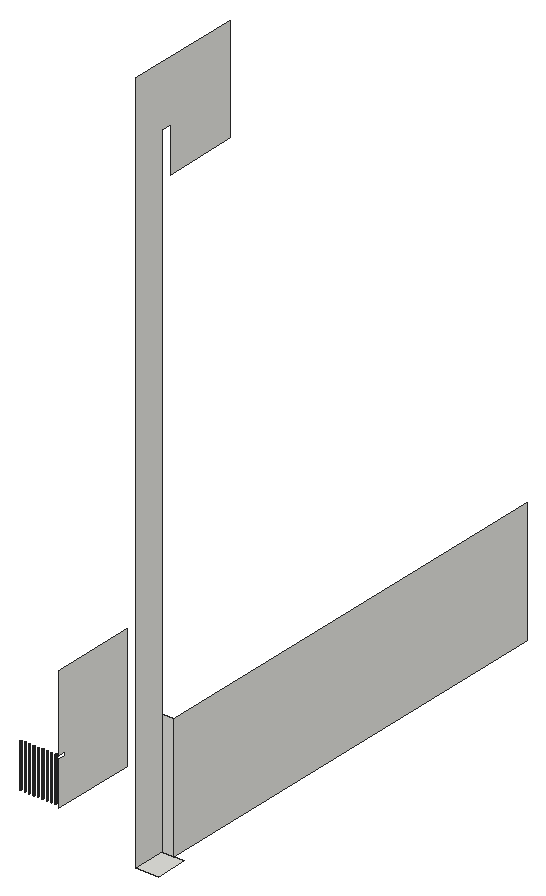
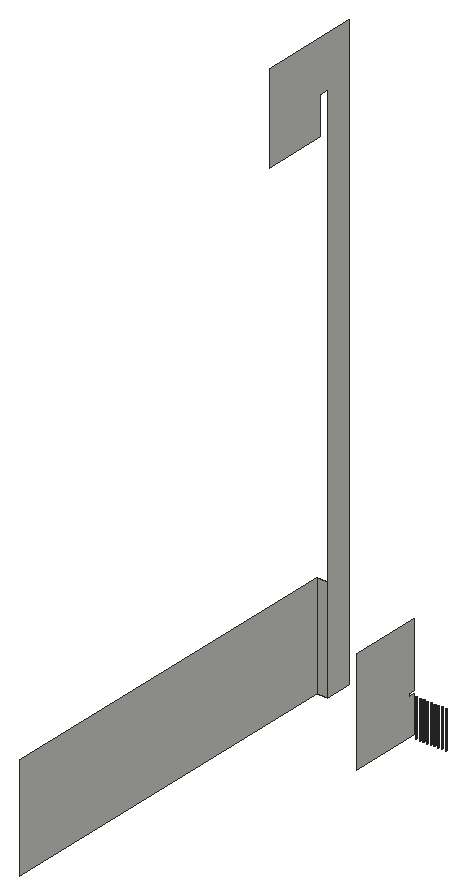
# SketchUp Ruby script. Lengths in inches.
U = 1.inch
M = Sketchup.active_model
def pt(a) = Geom::Point3d.new(a.map { |v| v * U })
def face(e, loops, mat)
  f = e.add_face(loops[0].map { |a| pt(a) })
  loops[1..].each { |l| e.add_face(l.map { |a| pt(a) }).erase! }
  f.material = f.back_material = mat if mat
  f
end
# faces: each face lists its corners as indices into pts; further lists are holes
def faces(e, pts, list, mat = nil) = list.each { |f| face(e, (f[0].is_a?(Array) ? f : [f]).map { |l| l.map { |i| pts[i] } }, mat) }
# xy, xz, yz: faces in a plane at the given z, y or x. An outline is a flat list of corners, or four numbers for a rectangle; further outlines are holes
def ring(l) = l.size == 4 ? [[l[0], l[1]], [l[2], l[1]], [l[2], l[3]], [l[0], l[3]]] : l.each_slice(2).to_a
def flat(e, list, mat, &to3) = list.each { |f| face(e, (f[0].is_a?(Array) ? f : [f]).map { |l| ring(l).map { |u, v| to3.(u, v) } }, mat) }
def xy(e, z, list, mat = nil) = flat(e, list, mat) { |x, y| [x, y, z] }
def xz(e, y, list, mat = nil) = flat(e, list, mat) { |x, z| [x, y, z] }
def yz(e, x, list, mat = nil) = flat(e, list, mat) { |y, z| [x, y, z] }
def lines(e, pts, list) = list.each { |a, b| e.add_line(pt(pts[a]), pt(pts[b])) }
# prism: a flat outline (further loops are holes) pulled along v
def prism(e, loops, v, mat = nil)
  f = face(e, loops, mat); d = Geom::Vector3d.new(v.map { |x| x * U })
  f.pushpull(f.normal.samedirection?(d) ? d.length : -d.length)
end
def box(e, o, s, mat = nil) = prism(e, [[o, [o[0] + s[0], o[1], o[2]], [o[0] + s[0], o[1] + s[1], o[2]], [o[0], o[1] + s[1], o[2]]]], [0, 0, s[2]], mat)
def at(x, y, z, deg = 0) = Geom::Transformation.translation(pt([x, y, z])) * Geom::Transformation.rotation(ORIGIN, Z_AXIS, deg.degrees)
def axes(o, x, y, z) = Geom::Transformation.new([*x, 0, *y, 0, *z, 0, *pt(o).to_a, 1])
def part(name) = M.definitions.add(name)
# library, detail: a bought-in or finely detailed component or shape, given as its bounding box
def library(name, o, s) = part(name).tap { |d| box(d.entities, o, s) }
def detail(e, o, s) = box(e.add_group.entities, o, s)
def put(e, d, t, mat = nil) = e.add_instance(d, t).tap { |i| i.material = mat if mat }
def group(e, t, mat = nil) = e.add_group.tap { |g| g.transformation = t; g.material = mat if mat }.entities
root = M.entities
xy(root,204.9375,[[673.48,81.125,703.6875,124.5],[472.27,135.31,472.06,135.34,471.86,135.42,471.69,135.55,471.5625,135.72,471.48,135.91,471.45,136.12,471.48,136.33,471.5625,136.53,471.69,136.7,471.86,136.83,472.06,136.91,472.27,136.93,472.48,136.91,472.67,136.83,472.84,136.7,472.97,136.53,473.05,136.33,473.08,136.12,473.05,135.91,472.97,135.72,472.84,135.55,472.67,135.42,472.48,135.34],[478.27,135.31,478.06,135.34,477.86,135.42,477.69,135.55,477.5625,135.72,477.48,135.91,477.45,136.12,477.48,136.33,477.5625,136.53,477.69,136.7,477.86,136.83,478.06,136.91,478.27,136.93,478.48,136.91,478.67,136.83,478.84,136.7,478.97,136.53,479.05,136.33,479.08,136.12,479.05,135.91,478.97,135.72,478.84,135.55,478.67,135.42,478.48,135.34],[484.2,135.31,483.99,135.34,483.8,135.42,483.63,135.55,483.5,135.72,483.42,135.91,483.39,136.12,483.42,136.33,483.5,136.53,483.63,136.7,483.8,136.83,483.99,136.91,484.2,136.93,484.41,136.91,484.61,136.83,484.78,136.7,484.91,136.53,484.99,136.33,485.02,136.12,484.99,135.91,484.91,135.72,484.78,135.55,484.61,135.42,484.41,135.34],[490.27,135.31,490.06,135.34,489.86,135.42,489.69,135.55,489.5625,135.72,489.48,135.91,489.45,136.12,489.48,136.33,489.5625,136.53,489.69,136.7,489.86,136.83,490.06,136.91,490.27,136.93,490.48,136.91,490.67,136.83,490.84,136.7,490.97,136.53,491.05,136.33,491.08,136.12,491.05,135.91,490.97,135.72,490.84,135.55,490.67,135.42,490.48,135.34],
  [496.27,135.31,496.06,135.34,495.86,135.42,495.69,135.55,495.5625,135.72,495.48,135.91,495.45,136.12,495.48,136.33,495.5625,136.53,495.69,136.7,495.86,136.83,496.06,136.91,496.27,136.93,496.48,136.91,496.67,136.83,496.84,136.7,496.97,136.53,497.05,136.33,497.08,136.12,497.05,135.91,496.97,135.72,496.84,135.55,496.67,135.42,496.48,135.34],[502.27,135.31,502.06,135.34,501.86,135.42,501.69,135.55,501.5625,135.72,501.48,135.91,501.45,136.12,501.48,136.33,501.5625,136.53,501.69,136.7,501.86,136.83,502.06,136.91,502.27,136.93,502.48,136.91,502.67,136.83,502.84,136.7,502.97,136.53,503.05,136.33,503.08,136.12,503.05,135.91,502.97,135.72,502.84,135.55,502.67,135.42,502.48,135.34],[508.14,135.31,507.93,135.34,507.74,135.42,507.57,135.55,507.4375,135.72,507.36,135.91,507.33,136.12,507.36,136.33,507.4375,136.53,507.57,136.7,507.74,136.83,507.93,136.91,508.14,136.93,508.35,136.91,508.55,136.83,508.72,136.7,508.85,136.53,508.93,136.33,508.95,136.12,508.93,135.91,508.85,135.72,508.72,135.55,508.55,135.42,508.35,135.34],[514.2,135.31,513.99,135.34,513.8,135.42,513.63,135.55,513.5,135.72,513.42,135.91,513.39,136.12,513.42,136.33,513.5,136.53,513.63,136.7,513.8,136.83,513.99,136.91,514.2,136.93,514.41,136.91,514.61,136.83,514.78,136.7,514.91,136.53,514.99,136.33,515.02,136.12,514.99,135.91,514.91,135.72,514.78,135.55,514.61,135.42,514.41,135.34],[520.27,135.31,520.06,135.34,519.86,135.42,519.69,135.55,519.5625,135.72,519.48,135.91,519.45,136.12,519.48,136.33,519.5625,136.53,519.69,136.7,519.86,136.83,520.06,136.91,520.27,136.93,520.48,136.91,520.67,136.83,520.84,136.7,520.97,136.53,521.05,136.33,521.08,136.12,521.05,135.91,520.97,135.72,520.84,135.55,520.67,135.42,520.48,135.34]])
xz(root,124.5,[[673.48,204.9375,690.4375,372.9375]])
yz(root,528.75,[[130.75,204.9375,130.75,264.83,140.05,264.83,140.05,269.02,130.75,269.02,130.75,372.9375,246,372.9375,246,204.9375]])
yz(root,673.48,[[81.125,204.9375,81.125,1168.125,241.25,1168.125,241.25,1024.6875,139.4375,1024.6875,139.4375,1085.75,124.5,1085.75,124.5,204.9375]])
yz(root,690.4375,[[124.5,204.9375,724.5,372.9375]])
p = [[471.86,135.42,204.9375],[472.06,135.34,204.9375],[472.06,135.34,264.83],[471.86,135.42,264.83],[472.27,135.31,204.9375],[472.27,135.31,264.83],
  [472.48,135.34,204.9375],[472.48,135.34,264.83],[472.67,135.42,204.9375],[472.67,135.42,264.83],[477.86,135.42,204.9375],[478.06,135.34,204.9375],
  [478.06,135.34,264.83],[477.86,135.42,264.83],[478.27,135.31,204.9375],[478.27,135.31,264.83],[478.48,135.34,204.9375],[478.48,135.34,264.83],
  [478.67,135.42,204.9375],[478.67,135.42,264.83],[483.8,135.42,204.9375],[483.99,135.34,204.9375],[483.99,135.34,264.83],[483.8,135.42,264.83],
  [484.2,135.31,204.9375],[484.2,135.31,264.83],[484.41,135.34,204.9375],[484.41,135.34,264.83],[484.61,135.42,204.9375],[484.61,135.42,264.83],
  [489.86,135.42,204.9375],[490.06,135.34,204.9375],[490.06,135.34,264.83],[489.86,135.42,264.83],[490.27,135.31,204.9375],[490.27,135.31,264.83],
  [490.48,135.34,204.9375],[490.48,135.34,264.83],[490.67,135.42,204.9375],[490.67,135.42,264.83],[495.86,135.42,204.9375],[496.06,135.34,204.9375],
  [496.06,135.34,264.83],[495.86,135.42,264.83],[496.27,135.31,204.9375],[496.27,135.31,264.83],[496.48,135.34,204.9375],[496.48,135.34,264.83],
  [496.67,135.42,204.9375],[496.67,135.42,264.83],[501.86,135.42,204.9375],[502.06,135.34,204.9375],[502.06,135.34,264.83],[501.86,135.42,264.83],
  [502.27,135.31,204.9375],[502.27,135.31,264.83],[502.48,135.34,204.9375],[502.48,135.34,264.83],[502.67,135.42,204.9375],[502.67,135.42,264.83],
  [507.74,135.42,204.9375],[507.93,135.34,204.9375],[507.93,135.34,264.83],[507.74,135.42,264.83],[508.14,135.31,204.9375],[508.14,135.31,264.83],
  [508.35,135.34,204.9375],[508.35,135.34,264.83],[508.55,135.42,204.9375],[508.55,135.42,264.83],[513.8,135.42,204.9375],[513.99,135.34,204.9375],
  [513.99,135.34,264.83],[513.8,135.42,264.83],[514.2,135.31,204.9375],[514.2,135.31,264.83],[514.41,135.34,204.9375],[514.41,135.34,264.83],
  [514.61,135.42,204.9375],[514.61,135.42,264.83],[519.86,135.42,204.9375],[520.06,135.34,204.9375],[520.06,135.34,264.83],[519.86,135.42,264.83],
  [520.27,135.31,204.9375],[520.27,135.31,264.83],[520.48,135.34,204.9375],[520.48,135.34,264.83],[520.67,135.42,204.9375],[520.67,135.42,264.83],
  [472.84,135.55,204.9375],[472.84,135.55,264.83],[477.69,135.55,204.9375],[477.69,135.55,264.83],[478.84,135.55,204.9375],[478.84,135.55,264.83],
  [483.63,135.55,204.9375],[483.63,135.55,264.83],[484.78,135.55,204.9375],[484.78,135.55,264.83],[489.69,135.55,204.9375],[489.69,135.55,264.83],
  [490.84,135.55,204.9375],[490.84,135.55,264.83],[495.69,135.55,204.9375],[495.69,135.55,264.83],[496.84,135.55,204.9375],[496.84,135.55,264.83],
  [501.69,135.55,204.9375],[501.69,135.55,264.83],[502.84,135.55,204.9375],[502.84,135.55,264.83],[507.57,135.55,204.9375],[507.57,135.55,264.83],
  [508.72,135.55,204.9375],[508.72,135.55,264.83],[513.63,135.55,204.9375],[513.63,135.55,264.83],[514.78,135.55,204.9375],[514.78,135.55,264.83],
  [519.69,135.55,204.9375],[519.69,135.55,264.83],[520.84,135.55,204.9375],[520.84,135.55,264.83],[472.97,135.72,204.9375],[472.97,135.72,264.83],
  [477.5625,135.72,204.9375],[477.5625,135.72,264.83],[478.97,135.72,204.9375],[478.97,135.72,264.83],[483.5,135.72,204.9375],[483.5,135.72,264.83],
  [484.91,135.72,204.9375],[484.91,135.72,264.83],[489.5625,135.72,204.9375],[489.5625,135.72,264.83],[490.97,135.72,204.9375],[490.97,135.72,264.83],
  [495.5625,135.72,204.9375],[495.5625,135.72,264.83],[496.97,135.72,204.9375],[496.97,135.72,264.83],[501.5625,135.72,204.9375],[501.5625,135.72,264.83],
  [502.97,135.72,204.9375],[502.97,135.72,264.83],[507.4375,135.72,204.9375],[507.4375,135.72,264.83],[508.85,135.72,204.9375],[508.85,135.72,264.83],
  [513.5,135.72,204.9375],[513.5,135.72,264.83],[514.91,135.72,204.9375],[514.91,135.72,264.83],[519.5625,135.72,204.9375],[519.5625,135.72,264.83],
  [520.97,135.72,204.9375],[520.97,135.72,264.83],[473.05,135.91,204.9375],[473.05,135.91,264.83],[477.48,135.91,204.9375],[477.48,135.91,264.83],
  [479.05,135.91,204.9375],[479.05,135.91,264.83],[483.42,135.91,204.9375],[483.42,135.91,264.83],[484.99,135.91,204.9375],[484.99,135.91,264.83],
  [489.48,135.91,204.9375],[489.48,135.91,264.83],[491.05,135.91,204.9375],[491.05,135.91,264.83],[495.48,135.91,204.9375],[495.48,135.91,264.83],
  [497.05,135.91,204.9375],[497.05,135.91,264.83],[501.48,135.91,204.9375],[501.48,135.91,264.83],[503.05,135.91,204.9375],[503.05,135.91,264.83],
  [507.36,135.91,204.9375],[507.36,135.91,264.83],[508.93,135.91,204.9375],[508.93,135.91,264.83],[513.42,135.91,204.9375],[513.42,135.91,264.83],
  [514.99,135.91,204.9375],[514.99,135.91,264.83],[519.48,135.91,204.9375],[519.48,135.91,264.83],[521.05,135.91,204.9375],[521.05,135.91,264.83],
  [473.08,136.12,204.9375],[473.08,136.12,264.83],[477.45,136.12,204.9375],[477.45,136.12,264.83],[479.08,136.12,204.9375],[479.08,136.12,264.83],
  [483.39,136.12,204.9375],[483.39,136.12,264.83],[485.02,136.12,204.9375],[485.02,136.12,264.83],[489.45,136.12,204.9375],[489.45,136.12,264.83],
  [491.08,136.12,204.9375],[491.08,136.12,264.83],[495.45,136.12,204.9375],[495.45,136.12,264.83],[497.08,136.12,204.9375],[497.08,136.12,264.83],
  [501.45,136.12,204.9375],[501.45,136.12,264.83],[503.08,136.12,204.9375],[503.08,136.12,264.83],[507.33,136.12,204.9375],[507.33,136.12,264.83],
  [508.95,136.12,204.9375],[508.95,136.12,264.83],[513.39,136.12,204.9375],[513.39,136.12,264.83],[515.02,136.12,204.9375],[515.02,136.12,264.83],
  [519.45,136.12,204.9375],[519.45,136.12,264.83],[521.08,136.12,204.9375],[521.08,136.12,264.83],[473.05,136.33,204.9375],[473.05,136.33,264.83],
  [477.48,136.33,204.9375],[477.48,136.33,264.83],[479.05,136.33,204.9375],[479.05,136.33,264.83],[483.42,136.33,204.9375],[483.42,136.33,264.83],
  [484.99,136.33,204.9375],[484.99,136.33,264.83],[489.48,136.33,204.9375],[489.48,136.33,264.83],[491.05,136.33,204.9375],[491.05,136.33,264.83],
  [495.48,136.33,204.9375],[495.48,136.33,264.83],[497.05,136.33,204.9375],[497.05,136.33,264.83],[501.48,136.33,204.9375],[501.48,136.33,264.83],
  [503.05,136.33,204.9375],[503.05,136.33,264.83],[507.36,136.33,204.9375],[507.36,136.33,264.83],[508.93,136.33,204.9375],[508.93,136.33,264.83],
  [513.42,136.33,204.9375],[513.42,136.33,264.83],[514.99,136.33,204.9375],[514.99,136.33,264.83],[519.48,136.33,204.9375],[519.48,136.33,264.83],
  [521.05,136.33,204.9375],[521.05,136.33,264.83],[472.97,136.53,204.9375],[472.97,136.53,264.83],[477.5625,136.53,204.9375],[477.5625,136.53,264.83],
  [478.97,136.53,204.9375],[478.97,136.53,264.83],[483.5,136.53,204.9375],[483.5,136.53,264.83],[484.91,136.53,204.9375],[484.91,136.53,264.83],
  [489.5625,136.53,204.9375],[489.5625,136.53,264.83],[490.97,136.53,204.9375],[490.97,136.53,264.83],[495.5625,136.53,204.9375],[495.5625,136.53,264.83],
  [496.97,136.53,204.9375],[496.97,136.53,264.83],[501.5625,136.53,204.9375],[501.5625,136.53,264.83],[502.97,136.53,204.9375],[502.97,136.53,264.83],
  [507.4375,136.53,204.9375],[507.4375,136.53,264.83],[508.85,136.53,204.9375],[508.85,136.53,264.83],[513.5,136.53,204.9375],[513.5,136.53,264.83],
  [514.91,136.53,204.9375],[514.91,136.53,264.83],[519.5625,136.53,204.9375],[519.5625,136.53,264.83],[520.97,136.53,204.9375],[520.97,136.53,264.83],
  [472.84,136.7,204.9375],[472.84,136.7,264.83],[477.69,136.7,204.9375],[477.69,136.7,264.83],[478.84,136.7,204.9375],[478.84,136.7,264.83],
  [483.63,136.7,204.9375],[483.63,136.7,264.83],[484.78,136.7,204.9375],[484.78,136.7,264.83],[489.69,136.7,204.9375],[489.69,136.7,264.83],
  [490.84,136.7,204.9375],[490.84,136.7,264.83],[495.69,136.7,204.9375],[495.69,136.7,264.83],[496.84,136.7,204.9375],[496.84,136.7,264.83],
  [501.69,136.7,204.9375],[501.69,136.7,264.83],[502.84,136.7,204.9375],[502.84,136.7,264.83],[507.57,136.7,204.9375],[507.57,136.7,264.83],
  [508.72,136.7,204.9375],[508.72,136.7,264.83],[513.63,136.7,204.9375],[513.63,136.7,264.83],[514.78,136.7,204.9375],[514.78,136.7,264.83],
  [519.69,136.7,204.9375],[519.69,136.7,264.83],[520.84,136.7,204.9375],[520.84,136.7,264.83],[472.67,136.83,204.9375],[472.67,136.83,264.83],
  [477.86,136.83,204.9375],[477.86,136.83,264.83],[478.67,136.83,204.9375],[478.67,136.83,264.83],[483.8,136.83,204.9375],[483.8,136.83,264.83],
  [484.61,136.83,204.9375],[484.61,136.83,264.83],[489.86,136.83,204.9375],[489.86,136.83,264.83],[490.67,136.83,204.9375],[490.67,136.83,264.83],
  [495.86,136.83,204.9375],[495.86,136.83,264.83],[496.67,136.83,204.9375],[496.67,136.83,264.83],[501.86,136.83,204.9375],[501.86,136.83,264.83],
  [502.67,136.83,204.9375],[502.67,136.83,264.83],[507.74,136.83,204.9375],[507.74,136.83,264.83],[508.55,136.83,204.9375],[508.55,136.83,264.83],
  [513.8,136.83,204.9375],[513.8,136.83,264.83],[514.61,136.83,204.9375],[514.61,136.83,264.83],[519.86,136.83,204.9375],[519.86,136.83,264.83],
  [520.67,136.83,204.9375],[520.67,136.83,264.83],[472.06,136.91,204.9375],[471.86,136.83,204.9375],[471.86,136.83,264.83],[472.06,136.91,264.83],
  [472.48,136.91,204.9375],[472.48,136.91,264.83],[478.06,136.91,204.9375],[478.06,136.91,264.83],[478.48,136.91,204.9375],[478.48,136.91,264.83],
  [483.99,136.91,204.9375],[483.99,136.91,264.83],[484.41,136.91,204.9375],[484.41,136.91,264.83],[490.06,136.91,204.9375],[490.06,136.91,264.83],
  [490.48,136.91,204.9375],[490.48,136.91,264.83],[496.06,136.91,204.9375],[496.06,136.91,264.83],[496.48,136.91,204.9375],[496.48,136.91,264.83],
  [502.06,136.91,204.9375],[502.06,136.91,264.83],[502.48,136.91,204.9375],[502.48,136.91,264.83],[507.93,136.91,204.9375],[507.93,136.91,264.83],
  [508.35,136.91,204.9375],[508.35,136.91,264.83],[513.99,136.91,204.9375],[513.99,136.91,264.83],[514.41,136.91,204.9375],[514.41,136.91,264.83],
  [520.06,136.91,204.9375],[520.06,136.91,264.83],[520.48,136.91,204.9375],[520.48,136.91,264.83],[472.27,136.93,204.9375],[472.27,136.93,264.83],
  [478.27,136.93,204.9375],[478.27,136.93,264.83],[484.2,136.93,204.9375],[484.2,136.93,264.83],[490.27,136.93,204.9375],[490.27,136.93,264.83],
  [496.27,136.93,204.9375],[496.27,136.93,264.83],[502.27,136.93,204.9375],[502.27,136.93,264.83],[508.14,136.93,204.9375],[508.14,136.93,264.83],
  [514.2,136.93,204.9375],[514.2,136.93,264.83],[520.27,136.93,204.9375],[520.27,136.93,264.83],[520.27,136.12,264.83],[520.27,136.12,204.9375],
  [514.27,136.12,264.83],[514.27,136.12,204.9375],[508.27,136.12,264.83],[508.27,136.12,204.9375],[502.27,136.12,264.83],[502.27,136.12,204.9375],
  [496.27,136.12,264.83],[496.27,136.12,204.9375],[490.27,136.12,264.83],[490.27,136.12,204.9375],[484.27,136.12,264.83],[484.27,136.12,204.9375],
  [478.27,136.12,264.83],[478.27,136.12,204.9375],[472.27,136.12,264.83],[472.27,136.12,204.9375]]
faces(root,p,[[0,1,2,3],[1,4,5,2],[4,6,7,5],[6,8,9,7],[10,11,12,13],[11,14,15,12],[14,16,17,15],[16,18,19,17],
  [20,21,22,23],[21,24,25,22],[24,26,27,25],[26,28,29,27],[30,31,32,33],[31,34,35,32],[34,36,37,35],[36,38,39,37],
  [40,41,42,43],[41,44,45,42],[44,46,47,45],[46,48,49,47],[50,51,52,53],[51,54,55,52],[54,56,57,55],[56,58,59,57],
  [60,61,62,63],[61,64,65,62],[64,66,67,65],[66,68,69,67],[70,71,72,73],[71,74,75,72],[74,76,77,75],[76,78,79,77],
  [80,81,82,83],[81,84,85,82],[84,86,87,85],[86,88,89,87],[8,90,91,9],[92,10,13,93],[18,94,95,19],[96,20,23,97],
  [28,98,99,29],[100,30,33,101],[38,102,103,39],[104,40,43,105],[48,106,107,49],[108,50,53,109],[58,110,111,59],[112,60,63,113],
  [68,114,115,69],[116,70,73,117],[78,118,119,79],[120,80,83,121],[88,122,123,89],[90,124,125,91],[126,92,93,127],[94,128,129,95],
  [130,96,97,131],[98,132,133,99],[134,100,101,135],[102,136,137,103],[138,104,105,139],[106,140,141,107],[142,108,109,143],[110,144,145,111],
  [146,112,113,147],[114,148,149,115],[150,116,117,151],[118,152,153,119],[154,120,121,155],[122,156,157,123],[124,158,159,125],[160,126,127,161],
  [128,162,163,129],[164,130,131,165],[132,166,167,133],[168,134,135,169],[136,170,171,137],[172,138,139,173],[140,174,175,141],[176,142,143,177],
  [144,178,179,145],[180,146,147,181],[148,182,183,149],[184,150,151,185],[152,186,187,153],[188,154,155,189],[156,190,191,157],[158,192,193,159],
  [194,160,161,195],[162,196,197,163],[198,164,165,199],[166,200,201,167],[202,168,169,203],[170,204,205,171],[206,172,173,207],[174,208,209,175],
  [210,176,177,211],[178,212,213,179],[214,180,181,215],[182,216,217,183],[218,184,185,219],[186,220,221,187],[222,188,189,223],[190,224,225,191],
  [192,226,227,193],[228,194,195,229],[196,230,231,197],[232,198,199,233],[200,234,235,201],[236,202,203,237],[204,238,239,205],[240,206,207,241],
  [208,242,243,209],[244,210,211,245],[212,246,247,213],[248,214,215,249],[216,250,251,217],[252,218,219,253],[220,254,255,221],[256,222,223,257],
  [224,258,259,225],[226,260,261,227],[262,228,229,263],[230,264,265,231],[266,232,233,267],[234,268,269,235],[270,236,237,271],[238,272,273,239],
  [274,240,241,275],[242,276,277,243],[278,244,245,279],[246,280,281,247],[282,248,249,283],[250,284,285,251],[286,252,253,287],[254,288,289,255],
  [290,256,257,291],[258,292,293,259],[260,294,295,261],[296,262,263,297],[264,298,299,265],[300,266,267,301],[268,302,303,269],[304,270,271,305],
  [272,306,307,273],[308,274,275,309],[276,310,311,277],[312,278,279,313],[280,314,315,281],[316,282,283,317],[284,318,319,285],[320,286,287,321],
  [288,322,323,289],[324,290,291,325],[292,326,327,293],[294,328,329,295],[330,296,297,331],[298,332,333,299],[334,300,301,335],[302,336,337,303],
  [338,304,305,339],[306,340,341,307],[342,308,309,343],[310,344,345,311],[346,312,313,347],[314,348,349,315],[350,316,317,351],[318,352,353,319],
  [354,320,321,355],[322,356,357,323],[358,324,325,359],[326,360,361,327],[362,363,364,365],[328,366,367,329],[368,330,331,369],[332,370,371,333],
  [372,334,335,373],[336,374,375,337],[376,338,339,377],[340,378,379,341],[380,342,343,381],[344,382,383,345],[384,346,347,385],[348,386,387,349],
  [388,350,351,389],[352,390,391,353],[392,354,355,393],[356,394,395,357],[396,358,359,397],[360,398,399,361],[400,362,365,401],[366,400,401,367],
  [402,368,369,403],[370,402,403,371],[404,372,373,405],[374,404,405,375],[406,376,377,407],[378,406,407,379],[408,380,381,409],[382,408,409,383],
  [410,384,385,411],[386,410,411,387],[412,388,389,413],[390,412,413,391],[414,392,393,415],[394,414,415,395],[416,396,397,417],[398,416,417,399]])
lines(root,p,[[418,419],[420,421],[422,423],[424,425],[426,427],[428,429],[430,431],[432,433],[434,435]])
